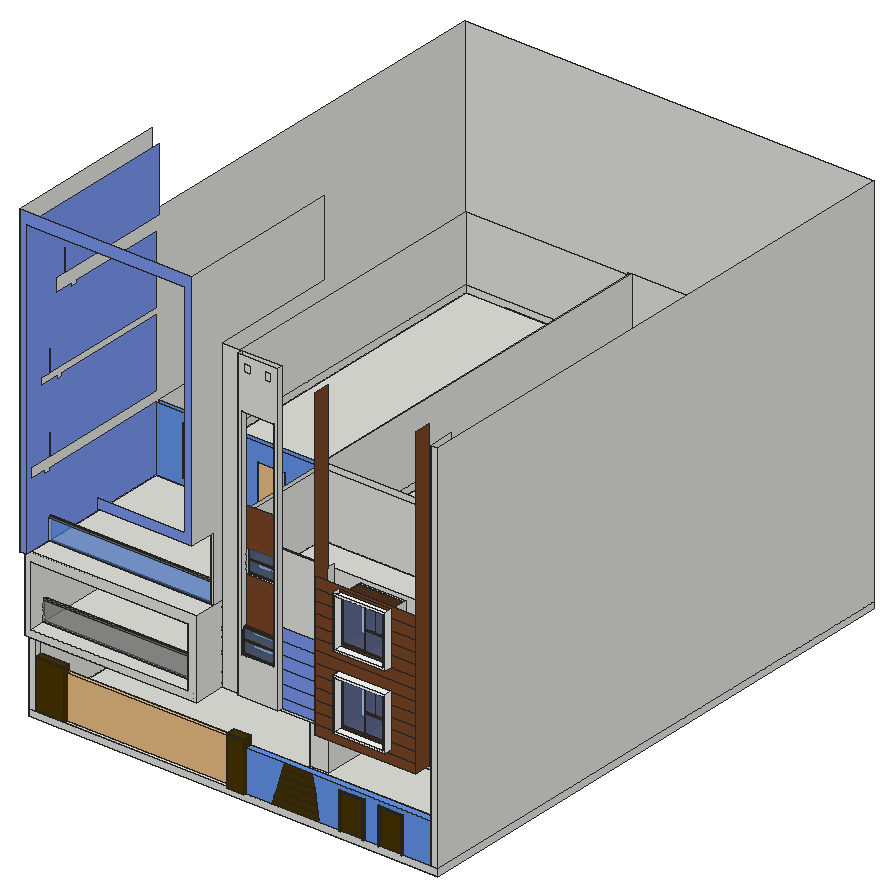
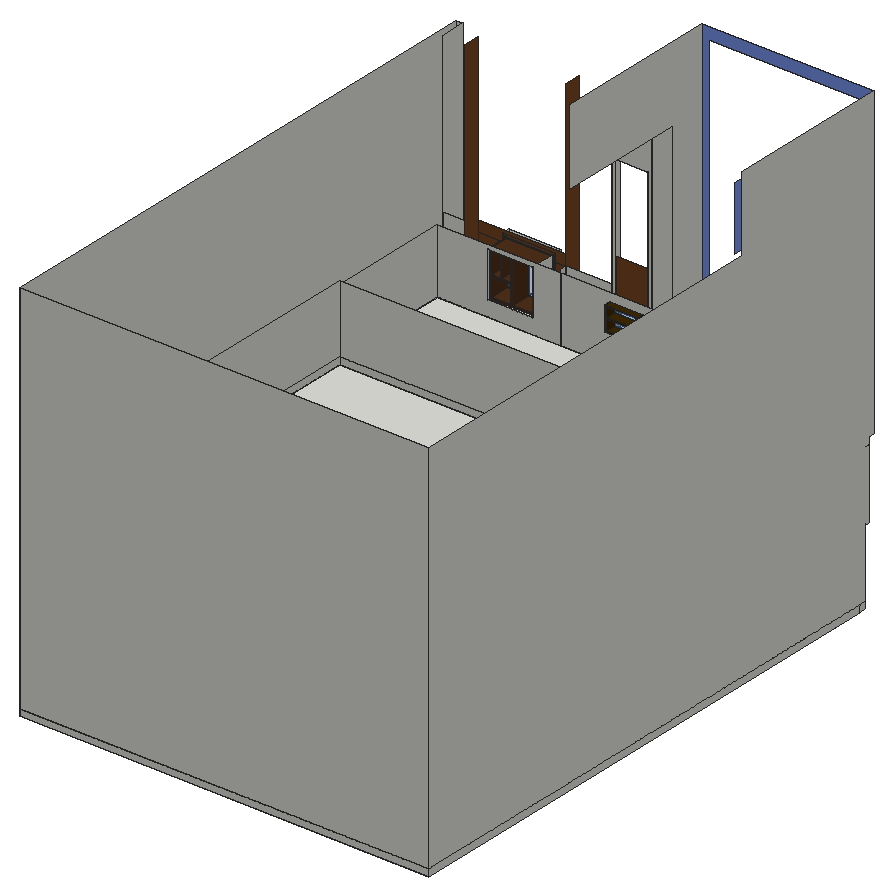
# SketchUp Ruby script. Lengths in inches.
U = 1.inch
M = Sketchup.active_model
def pt(a) = Geom::Point3d.new(a.map { |v| v * U })
def face(e, loops, mat)
  f = e.add_face(loops[0].map { |a| pt(a) })
  loops[1..].each { |l| e.add_face(l.map { |a| pt(a) }).erase! }
  f.material = f.back_material = mat if mat
  f
end
# faces: each face lists its corners as indices into pts; further lists are holes
def faces(e, pts, list, mat = nil) = list.each { |f| face(e, (f[0].is_a?(Array) ? f : [f]).map { |l| l.map { |i| pts[i] } }, mat) }
# xy, xz, yz: faces in a plane at the given z, y or x. An outline is a flat list of corners, or four numbers for a rectangle; further outlines are holes
def ring(l) = l.size == 4 ? [[l[0], l[1]], [l[2], l[1]], [l[2], l[3]], [l[0], l[3]]] : l.each_slice(2).to_a
def flat(e, list, mat, &to3) = list.each { |f| face(e, (f[0].is_a?(Array) ? f : [f]).map { |l| ring(l).map { |u, v| to3.(u, v) } }, mat) }
def xy(e, z, list, mat = nil) = flat(e, list, mat) { |x, y| [x, y, z] }
def xz(e, y, list, mat = nil) = flat(e, list, mat) { |x, z| [x, y, z] }
def yz(e, x, list, mat = nil) = flat(e, list, mat) { |y, z| [x, y, z] }
def lines(e, pts, list) = list.each { |a, b| e.add_line(pt(pts[a]), pt(pts[b])) }
# prism: a flat outline (further loops are holes) pulled along v
def prism(e, loops, v, mat = nil)
  f = face(e, loops, mat); d = Geom::Vector3d.new(v.map { |x| x * U })
  f.pushpull(f.normal.samedirection?(d) ? d.length : -d.length)
end
def box(e, o, s, mat = nil) = prism(e, [[o, [o[0] + s[0], o[1], o[2]], [o[0] + s[0], o[1] + s[1], o[2]], [o[0], o[1] + s[1], o[2]]]], [0, 0, s[2]], mat)
def at(x, y, z, deg = 0) = Geom::Transformation.translation(pt([x, y, z])) * Geom::Transformation.rotation(ORIGIN, Z_AXIS, deg.degrees)
def axes(o, x, y, z) = Geom::Transformation.new([*x, 0, *y, 0, *z, 0, *pt(o).to_a, 1])
def part(name) = M.definitions.add(name)
# library, detail: a bought-in or finely detailed component or shape, given as its bounding box
def library(name, o, s) = part(name).tap { |d| box(d.entities, o, s) }
def detail(e, o, s) = box(e.add_group.entities, o, s)
def put(e, d, t, mat = nil) = e.add_instance(d, t).tap { |i| i.material = mat if mat }
def group(e, t, mat = nil) = e.add_group.tap { |g| g.transformation = t; g.material = mat if mat }.entities
root = M.entities
M.materials.add("[0101_CornflowerBlue]").color = [121, 149, 237]
M.materials.add("[0101_CornflowerBlue]1").color = [100, 149, 237]
M.materials.add("[0117_GhostWhite]").color = [248, 248, 255]
M.materials.add("[Color C08]").color = [80, 48, 26]
M.materials.add("[Color C08]1").color = [63, 41, 0]
M.materials.add("[Color C08]2").color = [70, 51, 0]
M.materials.add("[Color C08]3").color = [73, 51, 0]
M.materials.add("[Color M00]").color = [255, 255, 255]
M.materials.add("[Metal Seamed]").color = [118, 119, 115]
M.materials.add("[Translucent Glass Blue]").color = [100, 149, 237]
M.materials["[Translucent Glass Blue]"].alpha = 0.5
M.materials.add("[Translucent Glass Gray]").color = [128, 128, 128]
M.materials["[Translucent Glass Gray]"].alpha = 0.5
M.materials.add("[Wood Veneer 01]").color = [120, 70, 37]
c1 = library("Group\#4",[0,0,0],[170.875,8.25,96.875])
c2 = part("Group\#3")
detail(c2.entities,[0,0,0],[48,6.625,84])
c3 = part("Group\#1")
xy(c3.entities,0,[[0,0,32.9375,6]],"[Color C08]")
xy(c3.entities,1.25,[[1.25,0,16.47,6],[17.37,0,31.6875,6]],"[Color C08]")
xy(c3.entities,14.6,[[17.37,0,31.6875,6]],"[Color C08]")
xy(c3.entities,15.72,[[17.37,0,24.18,6],[24.78,0,31.6875,6]],"[Color C08]")
xy(c3.entities,31.6875,[[1.25,0,16.47,6],[17.37,0,24.18,6],[24.78,0,31.6875,6]],"[Color C08]")
xy(c3.entities,32.9375,[[0,0,32.9375,6]],"[Color C08]")
xz(c3.entities,0,[[[0,0,32.9375,32.9375],[1.25,1.25,16.47,31.6875],[17.37,1.25,31.6875,14.6],[24.78,15.72,31.6875,31.6875],[17.37,15.72,24.18,31.6875]]],"[Color C08]")
xz(c3.entities,0,[[1.25,1.25,16.47,31.6875],[17.37,1.25,31.6875,14.6],[17.37,15.72,24.18,31.6875],[24.78,15.72,31.6875,31.6875]],"[Translucent Glass Blue]")
xz(c3.entities,6,[[[0,0,32.9375,32.9375],[1.25,1.25,16.47,31.6875],[17.37,1.25,31.6875,14.6],[24.78,15.72,31.6875,31.6875],[17.37,15.72,24.18,31.6875]]],"[Color C08]")
yz(c3.entities,0,[[0,0,6,32.9375]],"[Color C08]")
yz(c3.entities,1.25,[[0,1.25,6,31.6875]],"[Color C08]")
yz(c3.entities,16.47,[[0,1.25,6,31.6875]],"[Color C08]")
yz(c3.entities,17.37,[[0,1.25,6,14.6],[0,15.72,6,31.6875]],"[Color C08]")
yz(c3.entities,24.18,[[0,15.72,6,31.6875]],"[Color C08]")
yz(c3.entities,24.78,[[0,15.72,6,31.6875]],"[Color C08]")
yz(c3.entities,31.6875,[[0,1.25,6,14.6],[0,15.72,6,31.6875]],"[Color C08]")
yz(c3.entities,32.9375,[[0,0,6,32.9375]],"[Color C08]")
c4 = part("Group\#2")
xy(c4.entities,0,[[0,0,24.1875,6]])
xy(c4.entities,1.18,[[1.18,0,23.01,6]],"[Color C08]1")
xy(c4.entities,14.41,[[1.18,0,23.01,6]],"[Color C08]1")
xy(c4.entities,15.84,[[1.18,0,23.01,6]],"[Color C08]1")
xy(c4.entities,27.63,[[1.18,0,23.01,6]],"[Color C08]1")
xy(c4.entities,28.8125,[[0,0,24.1875,6]],"[Color C08]1")
xz(c4.entities,0,[[[0,0,24.1875,28.8125],[1.18,1.18,23.01,14.41],[1.18,15.84,23.01,27.63]]],"[Color C08]1")
xz(c4.entities,0,[[1.18,1.18,23.01,14.41],[1.18,15.84,23.01,27.63]],"[Translucent Glass Blue]")
xz(c4.entities,6,[[[0,0,24.1875,28.8125],[1.18,1.18,23.01,14.41],[1.18,15.84,23.01,27.63]]],"[Color C08]1")
yz(c4.entities,0,[[0,0,6,28.8125]],"[Color C08]1")
yz(c4.entities,1.18,[[0,1.18,6,14.41],[0,15.84,6,27.63]],"[Color C08]1")
yz(c4.entities,23.01,[[0,1.18,6,14.41],[0,15.84,6,27.63]],"[Color C08]1")
yz(c4.entities,24.1875,[[0,0,6,28.8125]],"[Color C08]1")
xy(root,-12,[[0,19.0625,720,31.0625],[0,31.0625,0,979.0625,720,979.0625,720,31.0625,708,31.0625,708,967.0625,12,967.0625,12,31.0625],[12,31.0625,708,967.0625]])
xy(root,0,[[352.24,15.9375,381.99,19.0625],[0,19.0625,0,979.0625,720,979.0625,720,19.0625,708,19.0625,708,967.0625,12,967.0625,12,19.0625],[12,19.0625,61.93,31.0625],[61.93,19.0625,352.24,31.0625],[352.24,19.0625,381.99,31.0625],
  [381.99,19.0625,708,31.0625],[[12,31.0625,708,967.0625],[401.48,422.71,435.98,512.27],[401.48,135.34,435.98,224.9]],[401.48,135.34,435.98,224.9]])
xy(root,0,[[548.19,17.125,550.43,19.0625],[589.04,17.125,591.29,19.0625],[616.89,17.125,618.5,19.0625],[657.11,17.125,658.72,19.0625]],"[Color C08]2")
xy(root,62.47,[[550.43,17.125,589.04,19.0625],[618.5,17.125,657.11,19.0625]],"[Color C08]2")
xy(root,64.08,[[616.89,17.125,658.72,19.0625]],"[Color C08]2")
xy(root,64.71,[[548.19,17.125,591.29,19.0625]],"[Color C08]2")
xy(root,72,[[381.99,19.0625,708,31.0625]],"[0101_CornflowerBlue]1")
xy(root,83.8125,[[352.24,15.9375,381.99,31.0625],[12,19.0625,61.93,31.0625]])
xy(root,86.8125,[[352.24,15.9375,381.99,31.0625],[12,19.0625,61.93,31.0625]],"[Color C08]3")
xy(root,120,[[0,9.875,12,19.0625],[12,9.875,12,967.0625,431.42,967.0625,297.1875,64.22,297.1875,9.875],[297.1875,9.875,303.1875,48.0625],[[297.1875,48.0625,297.1875,64.22,431.42,967.0625,708,967.0625,708,64.22,303.1875,64.22,303.1875,48.0625],[401.48,135.34,435.98,224.9]]])
xy(root,124,[[491.29,35.47,668.47,64.22],[338.82,55.09,410.48,64.22],[303.1875,75.64,708,284.375],[12,290.375,297.1875,967.0625],[[303.1875,290.375,708,967.0625],[401.48,422.71,435.98,512.27]]])
xy(root,132.5625,[[12,9.875,288.4375,36.0625],[12,36.0625,288.4375,40.0625],[288.4375,36.0625,297.1875,40.0625],[12,40.0625,288.4375,40.0625,288.4375,48.0625,297.1875,48.0625,297.1875,284.375,239.66,284.375,239.66,290.375,191.66,290.375,191.66,284.375,12,284.375],[288.4375,40.0625,297.1875,48.0625]])
xy(root,147.09,[[533.125,21.97,624.63,35.47]],"[Color M00]")
xy(root,147.8,[[65.42,280.375,135.92,284.375]],"[0117_GhostWhite]")
xy(root,150.65,[[536.9375,21.97,620.9375,35.47]],"[Color M00]")
xy(root,151.65,[[69.86,280.375,129.8,284.375]],"[0117_GhostWhite]")
xy(root,152.21,[[71.39,284.375,129.26,290.375]])
xy(root,153.16,[[539.1,35.47,618.73,75.64]])
xy(root,168.5625,[[12,36.0625,288.4375,40.0625]])
xy(root,171.5625,[[12,36.0625,288.4375,40.0625]],"[Metal Seamed]")
xy(root,191.01,[[346.17,55.09,403.55,64.22],[346.17,64.22,403.55,75.64]])
xy(root,208,[[191.66,284.375,239.66,290.375]])
xy(root,224.09,[[71.39,284.375,129.26,290.375]])
xy(root,224.92,[[69.86,280.375,129.8,284.375]],"[0117_GhostWhite]")
xy(root,230.05,[[65.42,280.375,135.92,284.375]],"[0117_GhostWhite]")
xy(root,232.79,[[539.1,35.47,618.73,75.64]])
xy(root,233.41,[[346.17,64.22,403.55,75.64]])
xy(root,235.46,[[536.9375,21.97,620.9375,35.47]],"[Color M00]")
xy(root,239.125,[[12,9.875,12,284.375,297.1875,284.375,297.1875,48.0625,288.4375,48.0625,288.4375,9.875]])
xy(root,239.34,[[533.125,21.97,624.63,35.47]],"[Color M00]")
xy(root,240,[[12,290.375,297.1875,967.0625]])
xy(root,244,[[12,290.375,297.1875,967.0625],[303.1875,290.375,708,967.0625]])
xy(root,250,[[303.1875,75.64,708,284.375]])
xy(root,256,[[0,0,12,9.875],[0,9.875,12,19.0625],[12,9.875,303.1875,48.0625],[12,52.0625,297.1875,284.375],[303.1875,75.64,708,284.375],
  [191.66,284.375,239.66,290.375]])
xy(root,270.59,[[62.16,280.375,138.1,284.375]],"[0117_GhostWhite]")
xy(root,276.84,[[533.125,21.97,624.63,35.47]],"[Color M00]")
xy(root,277.69,[[69.66,280.375,130.16,284.375]],"[0117_GhostWhite]")
xy(root,278.46,[[71.39,289.73,129.26,290.375]])
xy(root,278.46,[[70.47,284.375,71.39,289.73],[71.39,284.375,129.26,289.73]],"[Color C08]")
xy(root,280.4,[[536.9375,21.97,620.9375,35.47]],"[Color M00]")
xy(root,281.21,[[72.7,284.375,99.87,289.73],[101.47,284.375,127.03,289.73]],"[Color C08]")
xy(root,283.35,[[539.1,35.47,618.73,75.64]])
xy(root,292,[[12,48.0625,297.1875,52.0625]])
xy(root,295,[[12,48.0625,297.1875,52.0625]],"[Metal Seamed]")
xy(root,310.53,[[101.47,284.375,127.03,289.73]],"[Color C08]")
xy(root,313,[[101.47,284.375,113.63,289.73],[114.7,284.375,127.03,289.73]],"[Color C08]")
xy(root,313.44,[[346.17,64.22,403.55,75.64]])
xy(root,339.3125,[[191.66,284.375,239.66,290.375]])
xy(root,348.08,[[72.7,284.375,99.87,289.73],[101.47,284.375,113.63,289.73],[114.7,284.375,127.03,289.73]],"[Color C08]")
xy(root,350.34,[[71.39,284.375,129.26,290.375]])
xy(root,350.83,[[70.47,284.375,129.26,289.73]],"[Color C08]")
xy(root,351.78,[[69.66,280.375,130.16,284.375]],"[0117_GhostWhite]")
xy(root,355.83,[[346.17,64.22,403.55,75.64]])
xy(root,357.15,[[62.16,280.375,138.1,284.375]],"[0117_GhostWhite]")
xy(root,362.97,[[539.1,35.47,618.73,75.64]])
xy(root,365.21,[[536.9375,21.97,620.9375,35.47]],"[Color M00]")
xz(root,0,[[0,256,12,256,12,775.58,290.5625,775.58,290.5625,388,136.67,388,136.67,370.8125,303.1875,370.8125,303.1875,796.1875,0,796.1875]],"[0101_CornflowerBlue]")
xz(root,9.875,[[0,120,12,120,12,239.125,288.4375,239.125,288.4375,132.5625,12,132.5625,12,120,303.1875,120,303.1875,256,0,256]])
xz(root,15.9375,[[352.24,0,381.99,83.8125],[352.24,83.8125,381.99,86.8125]],"[Color C08]3")
xz(root,17.125,[[548.19,0,550.43,0,550.43,62.47,589.04,62.47,589.04,0,591.29,0,591.29,64.71,548.19,64.71],[616.89,0,618.5,0,618.5,62.47,657.11,62.47,657.11,0,658.72,0,658.72,64.08,616.89,64.08]],"[Color C08]2")
xz(root,19.0625,[[0,-12,720,0],[0,0,12,120],[708,0,720,663.5625]])
xz(root,19.0625,[[381.99,0,428.5625,0,432.375,12.3125,436.19,24.625,439.91,36.625,444.11,50.1875,447.69,61.75,450.87,72,381.99,72],[511.4375,0,548.19,0,548.19,64.71,591.29,64.71,591.29,0,616.89,0,616.89,64.08,658.72,64.08,658.72,0,708,0,708,72,499.48,72,501.18,61.75,503.1,50.1875,505.35,36.625,507.35,24.625,509.39,12.3125]],"[0101_CornflowerBlue]1")
xz(root,19.0625,[[428.5625,0,511.4375,0,509.39,12.3125,432.375,12.3125],[550.43,0,589.04,62.47],[618.5,0,657.11,62.47],[432.375,12.3125,509.39,12.3125,507.35,24.625,436.19,24.625],[436.19,24.625,507.35,24.625,505.35,36.625,439.91,36.625],
  [439.91,36.625,505.35,36.625,503.1,50.1875,444.11,50.1875],[444.11,50.1875,503.1,50.1875,501.18,61.75,447.69,61.75],[447.69,61.75,501.18,61.75,499.48,72,450.87,72]],"[Color C08]2")
xz(root,19.0625,[[12,0,61.93,83.8125],[12,83.8125,61.93,86.8125]],"[Color C08]3")
xz(root,21.97,[[[533.125,147.09,624.63,239.34],[536.9375,150.65,620.9375,235.46]],[[533.125,276.84,624.63,369.09],[536.9375,280.4,620.9375,365.21]]],"[Color M00]")
xz(root,31.0625,[[12,-12,708,0]])
xz(root,31.0625,[[381.99,0,708,72]],"[0101_CornflowerBlue]1")
xz(root,31.0625,[[12,0,61.93,83.8125],[352.24,0,381.99,83.8125],[12,83.8125,61.93,86.8125],[352.24,83.8125,381.99,86.8125]],"[Color C08]3")
xz(root,35.47,[[491.29,124,668.47,140.34],[491.29,140.34,668.47,140.34,668.47,159.84,624.63,159.84,624.63,147.09,533.125,147.09,533.125,159.84,491.29,159.84],[536.9375,150.65,620.9375,150.65,620.9375,159.84,618.73,159.84,618.73,153.16,539.1,153.16,539.1,159.84,536.9375,159.84],[491.29,159.84,533.125,179.34],[536.9375,159.84,539.1,179.34],
  [618.73,159.84,620.9375,179.34],[624.63,159.84,668.47,179.34],[491.29,179.34,533.125,198.84],[536.9375,179.34,539.1,198.84],[618.73,179.34,620.9375,198.84],
  [624.63,179.34,668.47,198.84],[491.29,198.84,533.125,218.34],[536.9375,198.84,539.1,218.34],[618.73,198.84,620.9375,218.34],[624.63,198.84,668.47,218.34],
  [491.29,218.34,533.125,237.84],[536.9375,218.34,539.1,218.34,539.1,232.79,618.73,232.79,618.73,218.34,620.9375,218.34,620.9375,235.46,536.9375,235.46],[624.63,218.34,668.47,237.84],[491.29,237.84,533.125,237.84,533.125,239.34,624.63,239.34,624.63,237.84,668.47,237.84,668.47,257.34,491.29,257.34],[491.29,257.34,668.47,276.84],
  [491.29,276.84,533.125,296.34],[[533.125,276.84,624.63,369.09],[536.9375,280.4,620.9375,365.21]],[624.63,276.84,668.47,296.34],[536.9375,280.4,620.9375,280.4,620.9375,296.34,618.73,296.34,618.73,283.35,539.1,283.35,539.1,296.34,536.9375,296.34],[491.29,296.34,533.125,315.84],
  [536.9375,296.34,539.1,315.84],[618.73,296.34,620.9375,315.84],[624.63,296.34,668.47,315.84],[491.29,315.84,533.125,335.34],[536.9375,315.84,539.1,335.34],
  [618.73,315.84,620.9375,335.34],[624.63,315.84,668.47,335.34],[491.29,335.34,533.125,354.84],[536.9375,335.34,539.1,354.84],[618.73,335.34,620.9375,354.84],
  [624.63,335.34,668.47,354.84],[491.29,354.84,533.125,354.84,533.125,369.09,624.63,369.09,624.63,354.84,668.47,354.84,668.47,374.34,491.29,374.34],[536.9375,354.84,539.1,354.84,539.1,362.97,618.73,362.97,618.73,354.84,620.9375,354.84,620.9375,365.21,536.9375,365.21]],"[Wood Veneer 01]")
xz(root,36.0625,[[12,168.5625,288.4375,171.5625]],"[Metal Seamed]")
xz(root,36.0625,[[12,132.5625,288.4375,168.5625]],"[Translucent Glass Gray]")
xz(root,40.0625,[[12,168.5625,288.4375,171.5625]],"[Metal Seamed]")
xz(root,40.0625,[[12,132.5625,288.4375,168.5625]],"[Translucent Glass Gray]")
xz(root,48.0625,[[288.4375,132.5625,297.1875,239.125],[297.1875,256,303.1875,370.8125]])
xz(root,48.0625,[[12,292,297.1875,295]],"[Metal Seamed]")
xz(root,48.0625,[[12,256,297.1875,292]],"[Translucent Glass Blue]")
xz(root,52.0625,[[12,292,297.1875,295]],"[Metal Seamed]")
xz(root,52.0625,[[12,256,297.1875,292]],"[Translucent Glass Blue]")
xz(root,55.09,[[[338.82,124,410.48,664],[346.17,191.01,403.55,575.64],[350.89,638.14,362.45,651.96],[386.39,638.14,397.95,651.96]]])
xz(root,64.22,[[303.1875,120,708,120,708,124,338.82,124,338.82,664,303.1875,664],[[338.82,124,410.48,664],[346.17,191.01,403.55,575.64]],[410.48,253.15,491.29,376.4],[668.47,257.72,708,384.85]])
xz(root,64.22,[[410.48,124,491.29,141.27],[668.47,124,708,143.97],[410.48,141.27,491.29,163.65],[668.47,143.97,708,163.97],[410.48,163.65,491.29,186.02],
  [668.47,163.97,708,182.72],[668.47,182.72,708,201.47],[410.48,186.02,491.29,208.4],[668.47,201.47,708,220.22],[410.48,208.4,491.29,230.77],
  [668.47,220.22,708,238.97],[410.48,230.77,491.29,253.15],[668.47,238.97,708,257.72]],"[0101_CornflowerBlue]")
xz(root,64.22,[[346.17,233.41,403.55,313.44],[346.17,355.83,403.55,423.38]],"[Wood Veneer 01]")
xz(root,75.64,[[[303.1875,124,491.29,250],[346.17,191.01,403.55,233.41]],[[491.29,124,708,244],[539.1,153.16,618.73,232.79]],[491.29,244,708,250],[303.1875,250,491.29,256],[491.29,250,708,256],
  [[303.1875,256,491.29,370],[346.17,313.44,403.55,355.83]],[[491.29,256,708,370],[539.1,283.35,618.73,362.97]]])
xz(root,135.34,[[401.48,0,435.98,120]])
xz(root,224.9,[[401.48,0,435.98,120]])
xz(root,280.375,[[[65.42,147.8,135.92,230.05],[69.86,151.65,129.8,224.92]],[[62.16,270.59,138.1,357.15],[69.66,277.69,130.16,351.78]]],"[0117_GhostWhite]")
xz(root,284.375,[[303.1875,124,708,244],[12,239.125,12,256,191.66,256,191.66,255.3125,239.66,255.3125,239.66,256,297.1875,256,297.1875,239.125],[303.1875,244,708,250],[303.1875,250,708,256],[191.66,255.3125,239.66,256],
  [303.1875,256,708,370]])
xz(root,284.375,[[[12,132.5625,191.66,132.5625,191.66,208,239.66,208,239.66,132.5625,297.1875,132.5625,297.1875,239.125,12,239.125],[65.42,147.8,135.92,230.05]],[[12,256,191.66,256,191.66,339.3125,239.66,339.3125,239.66,256,297.1875,256,297.1875,370.8125,12,370.8125],[62.16,270.59,138.1,357.15]]],"[0101_CornflowerBlue]1")
xz(root,284.375,[[[62.16,270.59,138.1,357.15],[69.66,277.69,130.16,351.78]]],"[0117_GhostWhite]")
xz(root,284.375,[[70.47,278.46,71.39,278.46,71.39,350.34,129.26,350.34,129.26,350.83,70.47,350.83],[[71.39,278.46,129.26,350.34],[72.7,281.21,99.87,348.08],[101.47,281.21,127.03,310.53],[114.7,313,127.03,348.08],[101.47,313,113.63,348.08]]],"[Color C08]")
xz(root,284.375,[[72.7,281.21,99.87,348.08],[101.47,281.21,127.03,310.53],[101.47,313,113.63,348.08],[114.7,313,127.03,348.08]],"[Translucent Glass Blue]")
xz(root,289.73,[[[70.47,278.46,129.26,350.83],[72.7,281.21,99.87,348.08],[101.47,281.21,127.03,310.53],[114.7,313,127.03,348.08],[101.47,313,113.63,348.08]]],"[Color C08]")
xz(root,290.375,[[191.66,124,239.66,132.5625],[303.1875,124,708,244],[12,240,297.1875,244],[12,244,297.1875,256],[303.1875,244,708,256],
  [303.1875,256,708,376]])
xz(root,290.375,[[[12,124,12,240,297.1875,240,297.1875,124,239.66,124,239.66,208,191.66,208,191.66,124],[71.39,152.21,129.26,224.09]],[[12,256,12,372,297.1875,372,297.1875,256,239.66,256,239.66,339.3125,191.66,339.3125,191.66,256],[71.39,278.46,129.26,350.34]]],"[0101_CornflowerBlue]1")
xz(root,422.71,[[401.48,0,435.98,124]])
xz(root,512.27,[[401.48,0,435.98,124]])
xz(root,967.0625,[[12,-12,708,0],[12,0,708,120],[12,124,297.1875,240],[297.1875,124,303.1875,244],[303.1875,124,708,244],
  [12,240,69.52,244],[69.52,240,81.15,244],[81.15,240,297.1875,244],[12,244,297.1875,256],[297.1875,244,303.1875,256],
  [303.1875,244,708,256],[12,256,297.1875,372],[297.1875,256,303.1875,376],[303.1875,256,708,376]])
xz(root,979.0625,[[0,-12,720,0],[0,0,720,663.5625]])
yz(root,0,[[19.0625,-12,31.0625,0],[31.0625,-12,979.0625,0],[19.0625,0,19.0625,120,9.875,120,9.875,256,0,256,0,796.1875,290.375,796.1875,290.375,664,979.0625,664,979.0625,0]])
yz(root,12,[[31.0625,-12,967.0625,0],[19.0625,0,31.0625,83.8125],[31.0625,0,967.0625,120],[19.0625,83.8125,31.0625,86.8125],[19.0625,86.8125,31.0625,120],
  [290.375,124,967.0625,240],[9.875,132.5625,36.0625,132.5625,36.0625,171.5625,40.0625,171.5625,40.0625,132.5625,284.375,132.5625,284.375,239.125,9.875,239.125],[36.0625,132.5625,40.0625,168.5625],[36.0625,168.5625,40.0625,171.5625],[19.0625,239.125,19.0625,256,48.0625,256,48.0625,292,52.0625,292,52.0625,256,284.375,256,284.375,239.125],
  [290.375,240,967.0625,244],[290.375,244,967.0625,256],[290.375,256,967.0625,372],[48.0625,292,52.0625,295]])
yz(root,12,[[0,256,48.0625,256,48.0625,295,52.0625,295,52.0625,256,284.375,256,284.375,370.8125,50.12,370.8125,50.12,365.8125,37.45,365.8125,37.45,370.8125,9.875,370.8125,9.875,388,48.0625,388,48.0625,427,52.0625,427,52.0625,388,284.375,388,284.375,508,77.9,508,77.9,503,65.23,503,65.23,508,31.0625,508,31.0625,520,48.0625,520,48.0625,559,52.0625,559,52.0625,520,284.375,520,284.375,640,110.4,640,110.4,635,97.73,635,97.73,640,64.22,640,64.22,664,81.22,664,81.22,703,85.22,703,85.22,663.5625,290.375,663.5625,290.375,775.58,0,775.58]],"[0101_CornflowerBlue]")
yz(root,61.93,[[19.0625,0,31.0625,83.8125],[19.0625,83.8125,31.0625,86.8125]],"[Color C08]3")
yz(root,62.16,[[280.375,270.59,284.375,357.15]],"[0117_GhostWhite]")
yz(root,65.42,[[280.375,147.8,284.375,230.05]],"[0117_GhostWhite]")
yz(root,69.66,[[280.375,277.69,284.375,351.78]],"[0117_GhostWhite]")
yz(root,69.86,[[280.375,151.65,284.375,224.92]],"[0117_GhostWhite]")
yz(root,70.47,[[284.375,278.46,289.73,350.83]],"[Color C08]")
yz(root,71.39,[[284.375,152.21,290.375,224.09],[284.375,278.46,290.375,350.34]])
yz(root,72.7,[[284.375,281.21,289.73,348.08]],"[Color C08]")
yz(root,99.87,[[284.375,281.21,289.73,348.08]],"[Color C08]")
yz(root,101.47,[[284.375,281.21,289.73,310.53],[284.375,313,289.73,348.08]],"[Color C08]")
yz(root,113.63,[[284.375,313,289.73,348.08]],"[Color C08]")
yz(root,114.7,[[284.375,313,289.73,348.08]],"[Color C08]")
yz(root,127.03,[[284.375,281.21,289.73,310.53],[284.375,313,289.73,348.08]],"[Color C08]")
yz(root,129.26,[[284.375,152.21,290.375,224.09],[284.375,278.46,289.73,350.34],[289.73,278.46,290.375,350.34]])
yz(root,129.26,[[284.375,350.34,289.73,350.83]],"[Color C08]")
yz(root,129.8,[[280.375,151.65,284.375,224.92]],"[0117_GhostWhite]")
yz(root,130.16,[[280.375,277.69,284.375,351.78]],"[0117_GhostWhite]")
yz(root,135.92,[[280.375,147.8,284.375,230.05]],"[0117_GhostWhite]")
yz(root,138.1,[[280.375,270.59,284.375,357.15]],"[0117_GhostWhite]")
yz(root,191.66,[[284.375,132.5625,290.375,208],[284.375,256,290.375,339.3125]])
yz(root,239.66,[[284.375,132.5625,290.375,208],[284.375,256,290.375,339.3125]])
yz(root,288.4375,[[9.875,132.5625,9.875,239.125,48.0625,239.125,48.0625,132.5625,40.0625,132.5625,40.0625,171.5625,36.0625,171.5625,36.0625,132.5625]])
yz(root,297.1875,[[290.375,124,967.0625,240],[48.0625,132.5625,284.375,239.125],[290.375,240,967.0625,244],[290.375,244,967.0625,256],[48.0625,256,52.0625,292],
  [52.0625,256,52.0625,295,48.0625,295,48.0625,365.8125,50.12,365.8125,50.12,370.8125,284.375,370.8125,284.375,256],[290.375,256,967.0625,372],[48.0625,292,52.0625,295]])
yz(root,303.1875,[[9.875,120,64.22,256],[64.22,124,75.64,244],[75.64,124,284.375,244],[290.375,124,967.0625,244],[64.22,244,75.64,256],
  [75.64,244,284.375,250],[290.375,244,967.0625,256],[75.64,250,83.7,256],[83.7,250,284.375,256],[48.0625,256,64.22,256,64.22,664,290.375,664,290.375,796.1875,0,796.1875,0,370.8125,48.0625,370.8125],
  [75.64,256,284.375,370],[290.375,256,967.0625,376]])
yz(root,338.82,[[55.09,124,64.22,664]])
yz(root,346.17,[[55.09,191.01,64.22,575.64],[64.22,191.01,75.64,233.41],[64.22,313.44,75.64,355.83]])
yz(root,352.24,[[15.9375,0,31.0625,83.8125],[15.9375,83.8125,31.0625,86.8125]],"[Color C08]3")
yz(root,381.99,[[19.0625,0,31.0625,72]])
yz(root,381.99,[[15.9375,0,19.0625,72],[15.9375,72,31.0625,83.8125],[15.9375,83.8125,31.0625,86.8125]],"[Color C08]3")
yz(root,401.48,[[135.34,0,224.9,120],[422.71,0,512.27,124]])
yz(root,403.55,[[55.09,191.01,64.22,575.64],[64.22,191.01,75.64,233.41],[64.22,313.44,75.64,355.83]])
yz(root,410.48,[[55.09,124,64.22,664]])
yz(root,435.98,[[135.34,0,224.9,120],[422.71,0,512.27,124]])
yz(root,491.29,[[64.22,124,75.64,244],[64.22,244,75.64,256],[64.22,256,75.64,376]])
yz(root,491.29,[[35.47,124,64.22,663.5625]],"[Wood Veneer 01]")
yz(root,533.125,[[21.97,147.09,35.47,239.34],[21.97,276.84,35.47,369.09]],"[Color M00]")
yz(root,536.9375,[[21.97,150.65,35.47,235.46],[21.97,280.4,35.47,365.21]],"[Color M00]")
yz(root,539.1,[[35.47,153.16,75.64,232.79],[35.47,283.35,75.64,362.97]])
yz(root,548.19,[[17.125,0,19.0625,64.71]],"[Color C08]2")
yz(root,550.43,[[17.125,0,19.0625,62.47]],"[Color C08]2")
yz(root,589.04,[[17.125,0,19.0625,62.47]],"[Color C08]2")
yz(root,591.29,[[17.125,0,19.0625,64.71]],"[Color C08]2")
yz(root,616.89,[[17.125,0,19.0625,64.08]],"[Color C08]2")
yz(root,618.5,[[17.125,0,19.0625,62.47]],"[Color C08]2")
yz(root,618.73,[[35.47,153.16,75.64,232.79],[35.47,283.35,75.64,362.97]])
yz(root,620.9375,[[21.97,150.65,35.47,235.46],[21.97,280.4,35.47,365.21]],"[Color M00]")
yz(root,624.63,[[21.97,147.09,35.47,239.34],[21.97,276.84,35.47,369.09]],"[Color M00]")
yz(root,657.11,[[17.125,0,19.0625,62.47]],"[Color C08]2")
yz(root,658.72,[[17.125,0,19.0625,64.08]],"[Color C08]2")
yz(root,668.47,[[35.47,124,64.22,663.5625]],"[Wood Veneer 01]")
yz(root,708,[[31.0625,-12,967.0625,0],[19.0625,0,31.0625,72],[31.0625,0,967.0625,120],[19.0625,72,31.0625,120],[19.0625,120,64.22,663.5625],
  [75.64,124,284.375,244],[290.375,124,967.0625,244],[75.64,244,284.375,250],[290.375,244,967.0625,256],[75.64,250,284.375,256],
  [75.64,256,284.375,370],[290.375,256,967.0625,376]])
yz(root,720,[[19.0625,-12,979.0625,0],[19.0625,0,979.0625,663.5625]])
p = [[297.1875,48.0625,124],[297.1875,9.875,124],[297.1875,48.0625,132.5625],[12,19.0625,244],[0,19.0625,244],[0,9.875,244],
  [0,19.0625,124],[0,19.0625,120],[297.1875,36.0625,132.5625],[297.1875,9.875,132.5625],[297.1875,48.0625,120]]
lines(root,p,[[0,1],[0,2],[3,4],[4,5],[6,7],[8,9],[0,10]])
put(root,c1,axes([61.93,25.64,0],[1.68509,0,0],[0,0.93,0],[0,0,0.7719]))
put(root,c2,axes([191.4,285.04,132.5625],[1.00545,0,0],[0,0.4897,0],[0,0,0.89807]))
put(root,c3,axes([70.47,283.69,152.21],[1.78505,0,0],[0,1.10259,0],[0,0,2.19699]))
put(root,c3,axes([539.1,35.47,153.16],[2.41746,0,0],[0,6.0075,0],[0,0,2.41746]))
put(root,c4,axes([346.22,58.39,191.01],[2.37,0,0],[0,2.8812,0],[0,0,1.47136]))
put(root,c2,axes([191.4,284.375,255.3125],[1.00545,0,0],[0,0.4897,0],[0,0,1]))
put(root,c3,axes([539.1,35.47,283.35],[2.41746,0,0],[0,6.0075,0],[0,0,2.41746]))
put(root,c4,axes([346.22,69.93,313.44],[2.37,0,0],[0,2.8812,0],[0,0,1.47136]))
